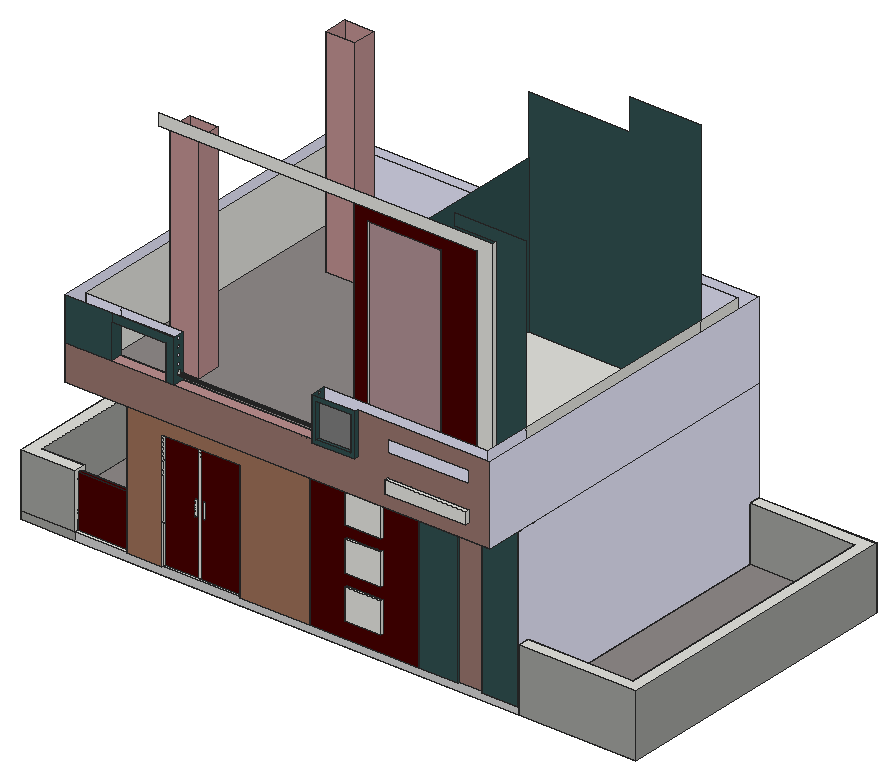
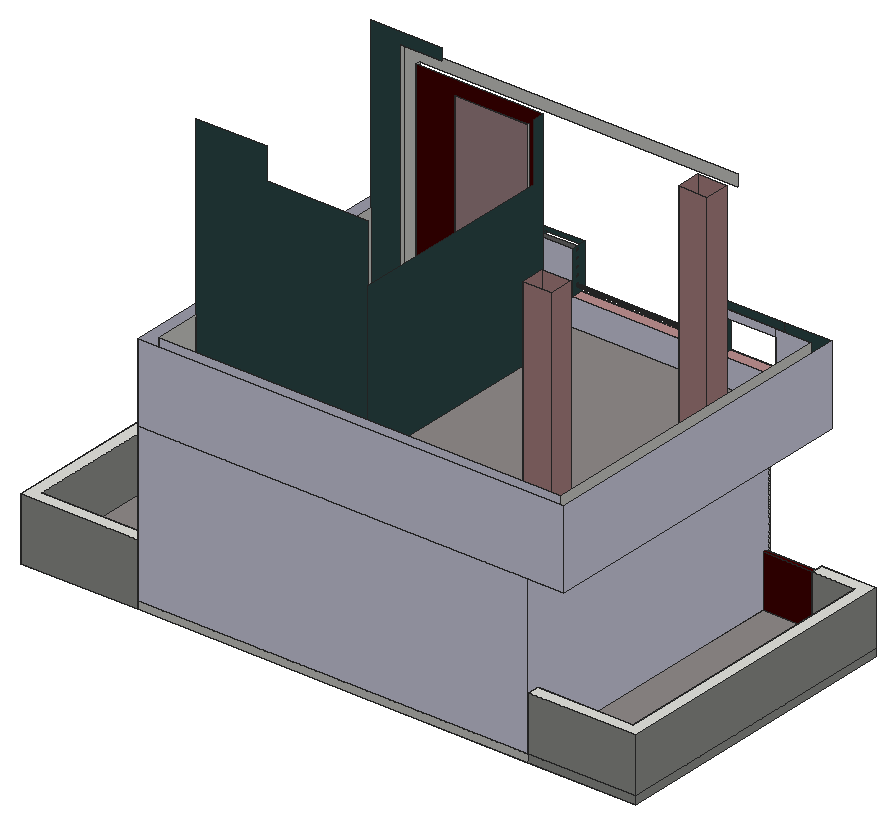
# SketchUp Ruby script. Lengths in inches.
U = 1.inch
M = Sketchup.active_model
def pt(a) = Geom::Point3d.new(a.map { |v| v * U })
def face(e, loops, mat)
  f = e.add_face(loops[0].map { |a| pt(a) })
  loops[1..].each { |l| e.add_face(l.map { |a| pt(a) }).erase! }
  f.material = f.back_material = mat if mat
  f
end
# faces: each face lists its corners as indices into pts; further lists are holes
def faces(e, pts, list, mat = nil) = list.each { |f| face(e, (f[0].is_a?(Array) ? f : [f]).map { |l| l.map { |i| pts[i] } }, mat) }
# xy, xz, yz: faces in a plane at the given z, y or x. An outline is a flat list of corners, or four numbers for a rectangle; further outlines are holes
def ring(l) = l.size == 4 ? [[l[0], l[1]], [l[2], l[1]], [l[2], l[3]], [l[0], l[3]]] : l.each_slice(2).to_a
def flat(e, list, mat, &to3) = list.each { |f| face(e, (f[0].is_a?(Array) ? f : [f]).map { |l| ring(l).map { |u, v| to3.(u, v) } }, mat) }
def xy(e, z, list, mat = nil) = flat(e, list, mat) { |x, y| [x, y, z] }
def xz(e, y, list, mat = nil) = flat(e, list, mat) { |x, z| [x, y, z] }
def yz(e, x, list, mat = nil) = flat(e, list, mat) { |y, z| [x, y, z] }
def lines(e, pts, list) = list.each { |a, b| e.add_line(pt(pts[a]), pt(pts[b])) }
# prism: a flat outline (further loops are holes) pulled along v
def prism(e, loops, v, mat = nil)
  f = face(e, loops, mat); d = Geom::Vector3d.new(v.map { |x| x * U })
  f.pushpull(f.normal.samedirection?(d) ? d.length : -d.length)
end
def box(e, o, s, mat = nil) = prism(e, [[o, [o[0] + s[0], o[1], o[2]], [o[0] + s[0], o[1] + s[1], o[2]], [o[0], o[1] + s[1], o[2]]]], [0, 0, s[2]], mat)
def at(x, y, z, deg = 0) = Geom::Transformation.translation(pt([x, y, z])) * Geom::Transformation.rotation(ORIGIN, Z_AXIS, deg.degrees)
def axes(o, x, y, z) = Geom::Transformation.new([*x, 0, *y, 0, *z, 0, *pt(o).to_a, 1])
def part(name) = M.definitions.add(name)
# library, detail: a bought-in or finely detailed component or shape, given as its bounding box
def library(name, o, s) = part(name).tap { |d| box(d.entities, o, s) }
def detail(e, o, s) = box(e.add_group.entities, o, s)
def put(e, d, t, mat = nil) = e.add_instance(d, t).tap { |i| i.material = mat if mat }
def group(e, t, mat = nil) = e.add_group.tap { |g| g.transformation = t; g.material = mat if mat }.entities
root = M.entities
M.materials.add("[0022_Maroon]").color = [71, 0, 0]
M.materials.add("[0040_Peru]").color = [150, 115, 108]
M.materials.add("[0078_DarkSlateGray]").color = [47, 79, 79]
M.materials.add("[0116_Lavender]").color = [230, 230, 250]
M.materials.add("[0118_Thistle]").color = [216, 191, 216]
M.materials.add("[0119_RosyBrown]").color = [188, 143, 143]
M.materials.add("[Carrera Marble]").color = [207, 207, 207]
M.materials.add("[Checker Plate]").color = [173, 142, 146]
M.materials.add("[Cladding Siding Tan]").color = [155, 110, 87]
M.materials.add("[Concrete Block 8x8 Gray]").color = [159, 160, 156]
M.materials.add("[Crushed Rock Gravel]").color = [124, 124, 124]
M.materials.add("[Stone Marble]").color = [143, 138, 136]
xy(root,0,[[0,60,165,522],[165,60,765,522],[765,60,945,522]])
xy(root,12,[[165,58,218.1875,60],[338.1875,58,446.1875,60],[446.1875,58,614.1875,60],[0,60,0,522,165,522,165,504,18,504,18,78,84,78,84,60],[84,60,165,65.6],
  [165,60,165,210,183,210,183,78,218.1875,78,218.1875,60],[338.1875,60,338.1875,78,747,78,747,210,765,210,765,60],[218.1875,64.63,338.1875,73.27],[84,65.6,165,71.35],[218.1875,73.27,338.1875,78],
  [183,78,747,210],[165,210,291.55,222],[291.55,210,388.24,214.18],[388.24,210,765,222],[291.55,214.18,388.24,218.54],
  [291.55,218.54,388.24,222],[165,222,165,522,765,522,765,222,753,222,753,321,527.52,321,527.52,330,600,330,600,432.82,609,432.82,609,330,753,330,753,510,609,510,609,487.39,600,487.39,600,510,366,510,366,330,454.54,330,454.54,321,258.23,321,258.23,330,357,330,357,510,177,510,177,330,199.29,330,199.29,321,177,321,177,222],[177,222,753,222,753,321,527.52,321,527.52,330,454.54,330,454.54,321,258.23,321,258.23,330,199.29,330,199.29,321,177,321],[177,330,357,510],[366,330,600,330,600,432.82,609,432.82,609,487.39,600,487.39,600,510,366,510],
  [609,330,753,510]])
xy(root,12,[[614.1875,58,674.1875,60],[710.1875,58,765,60]],"[0078_DarkSlateGray]")
xy(root,12,[[218.1875,60,338.1875,64.63]],"[Carrera Marble]")
xy(root,12,[[84,71.35,165,71.35,165,504,18,504,18,78,84,78],[765,78,927,504]],"[Stone Marble]")
xy(root,38.73,[[503.09,55,557.71,58]])
xy(root,86.3,[[503.09,55,557.71,58]])
xy(root,92.125,[[84,65.6,165,71.35]],"[0022_Maroon]")
xy(root,96,[[0,60,84,60,84,78,18,78,18,504,165,504,165,522,0,522],[765,60,945,60,945,522,765,522,765,504,927,504,927,78,765,78]])
xy(root,105.11,[[503.09,55,557.71,58]])
xy(root,142.5,[[600,432.82,609,487.39]])
xy(root,152.67,[[503.09,55,557.71,58]])
xy(root,157,[[199.29,321,258.23,330],[454.54,321,527.52,330]])
xy(root,168.44,[[291.55,210,388.24,214.18],[291.55,214.18,388.24,218.54],[291.55,218.54,388.24,222]])
xy(root,171.67,[[503.09,55,557.71,58]])
xy(root,193.9375,[[218.1875,58,338.1875,60],[218.1875,60,338.1875,64.63],[218.1875,64.63,338.1875,73.27],[218.1875,73.27,338.1875,78]])
xy(root,219.23,[[503.09,55,557.71,58]])
xy(root,252,[[139.72,26.33,136.64,26.86,133.79,28.17,131.38,30.17,129.58,32.73,128.49,35.67,128.21,38.79,128.74,41.88,130.05,44.72,132.06,47.13,134.62,48.9375,137.56,50.02,140.68,50.31,143.76,49.77,146.61,48.46,149.01,46.46,150.82,43.9,151.9,40.96,152.19,37.84,151.66,34.75,150.35,31.91,148.34,29.5,145.78,27.69,142.84,26.61],[230.54,26.33,227.45,26.86,224.6,28.17,222.2,30.17,220.39,32.73,219.31,35.67,219.02,38.79,219.55,41.88,220.87,44.72,222.87,47.13,225.43,48.9375,228.37,50.02,231.49,50.31,234.58,49.77,237.42,48.46,239.83,46.46,241.63,43.9,242.72,40.96,243,37.84,242.47,34.75,241.16,31.91,239.15,29.5,236.6,27.69,233.66,26.61],[333.47,26.33,330.39,26.86,327.54,28.17,325.13,30.17,323.33,32.73,322.24,35.67,321.96,38.79,322.49,41.88,323.8,44.72,325.81,47.13,328.37,48.9375,331.31,50.02,334.43,50.31,337.51,49.77,340.36,48.46,342.76,46.46,344.57,43.9,345.65,40.96,345.94,37.84,345.41,34.75,344.1,31.91,342.09,29.5,339.53,27.69,336.59,26.61],[453.47,26.33,450.39,26.86,447.54,28.17,445.13,30.17,443.33,32.73,442.24,35.67,441.96,38.79,442.49,41.88,443.8,44.72,445.81,47.13,448.37,48.9375,451.31,50.02,454.43,50.31,457.51,49.77,460.36,48.46,462.76,46.46,464.57,43.9,465.65,40.96,465.94,37.84,465.41,34.75,464.1,31.91,462.09,29.5,459.53,27.69,456.59,26.61],[573.47,26.33,570.39,26.86,567.54,28.17,565.13,30.17,563.33,32.73,562.24,35.67,561.96,38.79,562.49,41.88,563.8,44.72,565.81,47.13,568.37,48.9375,571.31,50.02,574.43,50.31,577.51,49.77,580.36,48.46,582.76,46.46,584.57,43.9,585.65,40.96,585.94,37.84,585.41,34.75,584.1,31.91,582.09,29.5,579.53,27.69,576.59,26.61],
  [693.47,26.33,690.39,26.86,687.54,28.17,685.13,30.17,683.33,32.73,682.24,35.67,681.96,38.79,682.49,41.88,683.8,44.72,685.81,47.13,688.37,48.9375,691.31,50.02,694.43,50.31,697.51,49.77,700.36,48.46,702.76,46.46,704.57,43.9,705.65,40.96,705.94,37.84,705.41,34.75,704.1,31.91,702.09,29.5,699.53,27.69,696.59,26.61],[165,58,218.1875,60],[218.1875,58,338.1875,60],[338.1875,58,446.1875,60],[446.1875,58,614.1875,60],
  [614.1875,58,674.1875,60],[710.1875,58,765,60],[165,60,165,210,183,210,183,78,218.1875,78,218.1875,60],[218.1875,60,338.1875,78],[338.1875,60,338.1875,78,747,78,747,210,765,210,765,60],
  [183,78,747,210],[136.96,95.37,133.87,95.86,131.01,97.13,128.57,99.11,126.73,101.64,125.61,104.57,125.29,107.68,125.78,110.78,127.05,113.64,129.03,116.07,131.5625,117.91,134.49,119.03,137.6,119.36,140.7,118.86,143.56,117.59,145.99,115.62,147.83,113.08,148.95,110.15,149.28,107.04,148.79,103.95,147.51,101.08,145.54,98.65,143,96.8125,140.08,95.69],[165,210,765,222],[136.96,215.37,133.87,215.86,131.01,217.13,128.57,219.11,126.73,221.64,125.61,224.57,125.29,227.68,125.78,230.78,127.05,233.64,129.03,236.07,131.5625,237.91,134.49,239.03,137.6,239.36,140.7,238.86,143.56,237.59,145.99,235.62,147.83,233.08,148.95,230.15,149.28,227.04,148.79,223.95,147.51,221.08,145.54,218.65,143,216.8125,140.08,215.69],[165,222,165,522,765,522,765,222,753,222,753,321,609,321,609,330,753,330,753,510,609,510,609,321,600,321,600,510,366,510,366,321,357,321,357,510,177,510,177,330,357,330,357,321,177,321,177,222],
  [177,222,177,321,357,321,357,330,177,330,177,510,357,510,357,321,366,321,366,510,600,510,600,321,609,321,609,510,753,510,753,330,609,330,609,321,753,321,753,222],[366,321,600,330],[136.96,335.37,133.87,335.86,131.01,337.13,128.57,339.11,126.73,341.64,125.61,344.57,125.29,347.68,125.78,350.78,127.05,353.64,129.03,356.07,131.5625,357.91,134.49,359.03,137.6,359.36,140.7,358.86,143.56,357.59,145.99,355.62,147.83,353.08,148.95,350.15,149.28,347.04,148.79,343.95,147.51,341.08,145.54,338.65,143,336.8125,140.08,335.69],[136.96,455.37,133.87,455.86,131.01,457.13,128.57,459.11,126.73,461.64,125.61,464.57,125.29,467.68,125.78,470.78,127.05,473.64,129.03,476.07,131.5625,477.91,134.49,479.03,137.6,479.36,140.7,478.86,143.56,477.59,145.99,475.62,147.83,473.08,148.95,470.15,149.28,467.04,148.79,463.95,147.51,461.08,145.54,458.65,143,456.8125,140.08,455.69]])
xy(root,252,[[[111,6,111,522,165,522,165,58,674.1875,58,674.1875,60,710.1875,60,710.1875,58,765,58,765,6],[136.96,335.37,140.08,335.69,143,336.8125,145.54,338.65,147.51,341.08,148.79,343.95,149.28,347.04,148.95,350.15,147.83,353.08,145.99,355.62,143.56,357.59,140.7,358.86,137.6,359.36,134.49,359.03,131.5625,357.91,129.03,356.07,127.05,353.64,125.78,350.78,125.29,347.68,125.61,344.57,126.73,341.64,128.57,339.11,131.01,337.13,133.87,335.86],[136.96,215.37,140.08,215.69,143,216.8125,145.54,218.65,147.51,221.08,148.79,223.95,149.28,227.04,148.95,230.15,147.83,233.08,145.99,235.62,143.56,237.59,140.7,238.86,137.6,239.36,134.49,239.03,131.5625,237.91,129.03,236.07,127.05,233.64,125.78,230.78,125.29,227.68,125.61,224.57,126.73,221.64,128.57,219.11,131.01,217.13,133.87,215.86],[136.96,95.37,140.08,95.69,143,96.8125,145.54,98.65,147.51,101.08,148.79,103.95,149.28,107.04,148.95,110.15,147.83,113.08,145.99,115.62,143.56,117.59,140.7,118.86,137.6,119.36,134.49,119.03,131.5625,117.91,129.03,116.07,127.05,113.64,125.78,110.78,125.29,107.68,125.61,104.57,126.73,101.64,128.57,99.11,131.01,97.13,133.87,95.86],[230.54,26.33,233.66,26.61,236.6,27.69,239.15,29.5,241.16,31.91,242.47,34.75,243,37.84,242.72,40.96,241.63,43.9,239.83,46.46,237.42,48.46,234.58,49.77,231.49,50.31,228.37,50.02,225.43,48.9375,222.87,47.13,220.87,44.72,219.55,41.88,219.02,38.79,219.31,35.67,220.39,32.73,222.2,30.17,224.6,28.17,227.45,26.86],[333.47,26.33,336.59,26.61,339.53,27.69,342.09,29.5,344.1,31.91,345.41,34.75,345.94,37.84,345.65,40.96,344.57,43.9,342.76,46.46,340.36,48.46,337.51,49.77,334.43,50.31,331.31,50.02,328.37,48.9375,325.81,47.13,323.8,44.72,322.49,41.88,321.96,38.79,322.24,35.67,323.33,32.73,325.13,30.17,327.54,28.17,330.39,26.86],[453.47,26.33,456.59,26.61,459.53,27.69,462.09,29.5,464.1,31.91,465.41,34.75,465.94,37.84,465.65,40.96,464.57,43.9,462.76,46.46,460.36,48.46,457.51,49.77,454.43,50.31,451.31,50.02,448.37,48.9375,445.81,47.13,443.8,44.72,442.49,41.88,441.96,38.79,442.24,35.67,443.33,32.73,445.13,30.17,447.54,28.17,450.39,26.86],[573.47,26.33,576.59,26.61,579.53,27.69,582.09,29.5,584.1,31.91,585.41,34.75,585.94,37.84,585.65,40.96,584.57,43.9,582.76,46.46,580.36,48.46,577.51,49.77,574.43,50.31,571.31,50.02,568.37,48.9375,565.81,47.13,563.8,44.72,562.49,41.88,561.96,38.79,562.24,35.67,563.33,32.73,565.13,30.17,567.54,28.17,570.39,26.86],[693.47,26.33,696.59,26.61,699.53,27.69,702.09,29.5,704.1,31.91,705.41,34.75,705.94,37.84,705.65,40.96,704.57,43.9,702.76,46.46,700.36,48.46,697.51,49.77,694.43,50.31,691.31,50.02,688.37,48.9375,685.81,47.13,683.8,44.72,682.49,41.88,681.96,38.79,682.24,35.67,683.33,32.73,685.13,30.17,687.54,28.17,690.39,26.86],[139.72,26.33,142.84,26.61,145.78,27.69,148.34,29.5,150.35,31.91,151.66,34.75,152.19,37.84,151.9,40.96,150.82,43.9,149.01,46.46,146.61,48.46,143.76,49.77,140.68,50.31,137.56,50.02,134.62,48.9375,132.06,47.13,130.05,44.72,128.74,41.88,128.21,38.79,128.49,35.67,129.58,32.73,131.38,30.17,133.79,28.17,136.64,26.86],[136.96,455.37,140.08,455.69,143,456.8125,145.54,458.65,147.51,461.08,148.79,463.95,149.28,467.04,148.95,470.15,147.83,473.08,145.99,475.62,143.56,477.59,140.7,478.86,137.6,479.36,134.49,479.03,131.5625,477.91,129.03,476.07,127.05,473.64,125.78,470.78,125.29,467.68,125.61,464.57,126.73,461.64,128.57,459.11,131.01,457.13,133.87,455.86]]],"[0118_Thistle]")
xy(root,264,[[677.8125,90,677.8125,96,483,96,483,432,747,432,747,96,701.8125,96,701.8125,90],[201,96,245.25,133.3125],[201,394.6875,245.25,432]])
xy(root,264,[[[129,24,747,24,747,96,701.8125,96,701.8125,90,677.8125,90,677.8125,96,483,96,483,432,747,432,747,504,129,504],[201,394.6875,245.25,432],[201,96,245.25,133.3125]]],"[Stone Marble]")
xy(root,275.13,[[607.99,0,731.55,6]])
xy(root,286.07,[[505.07,96,616.93,98]])
xy(root,294.2,[[607.99,0,731.55,6]])
xy(root,306,[[495,0,561,6],[267,6,279,24]])
xy(root,306,[[183,6,267,24],[279,6,495,24]],"[0119_RosyBrown]")
xy(root,312.125,[[501.125,0,554.875,6]],"[0078_DarkSlateGray]")
xz(root,0,[[607.99,275.13,731.55,294.2]])
xz(root,0,[[[495,306,561,372],[501.125,312.125,554.875,365.875]]],"[0078_DarkSlateGray]")
xz(root,6,[[607.99,275.13,731.55,294.2]])
xz(root,6,[[[111,252,765,252,765,372,561,372,561,306,111,306],[607.99,329.13,731.55,348.2],[607.99,275.13,731.55,294.2]]],"[0040_Peru]")
xz(root,6,[[111,306,183,372],[267,306,279,306,279,372,183,372,183,360,267,360]],"[0078_DarkSlateGray]")
xz(root,6,[[501.125,312.125,554.875,365.875]],"[Crushed Rock Gravel]")
xz(root,24,[[129,264,129,372,183,372,183,306,495,306,495,372,747,372,747,264],[267,306,267,360,183,360,183,372,279,372,279,306]],"[0116_Lavender]")
xz(root,55,[[503.09,38.73,557.71,86.3],[503.09,105.11,557.71,152.67],[503.09,171.67,557.71,219.23]])
xz(root,58,[[503.09,38.73,557.71,86.3],[503.09,105.11,557.71,152.67],[503.09,171.67,557.71,219.23]])
xz(root,58,[[[446.1875,12,614.1875,252],[503.09,171.67,557.71,219.23],[503.09,105.11,557.71,152.67],[503.09,38.73,557.71,86.3]]],"[0022_Maroon]")
xz(root,58,[[614.1875,12,674.1875,252],[710.1875,12,765,252]],"[0078_DarkSlateGray]")
xz(root,58,[[165,12,218.1875,12,218.1875,193.9375,338.1875,193.9375,338.1875,12,446.1875,12,446.1875,252,165,252]],"[Cladding Siding Tan]")
xz(root,60,[[165,12,165,252,446.1875,252,446.1875,12,338.1875,12,338.1875,193.9375,218.1875,193.9375,218.1875,12],[446.1875,12,614.1875,252],[614.1875,12,674.1875,252],[710.1875,12,765,252]])
xz(root,60,[[674.1875,12,710.1875,252]],"[0040_Peru]")
xz(root,60,[[84,0,765,12]],"[Carrera Marble]")
xz(root,60,[[0,0,84,12],[765,0,945,96],[0,12,84,96]],"[Concrete Block 8x8 Gray]")
xz(root,64.63,[[270.93,12,272.88,193.9375],[264.42,94.01,268.42,120.19],[276.42,94.01,280.42,120.19]])
xz(root,64.63,[[[218.1875,12,270.93,193.9375],[264.42,94.01,268.42,120.19]],[[272.88,12,338.1875,193.9375],[276.42,94.01,280.42,120.19]]],"[0022_Maroon]")
xz(root,65.6,[[84,12,165,92.125]],"[0022_Maroon]")
xz(root,71.35,[[84,12,165,92.125]],"[0022_Maroon]")
xz(root,73.27,[[218.1875,12,338.1875,193.9375]])
xz(root,78,[[183,12,218.1875,252],[338.1875,12,747,252],[218.1875,193.9375,338.1875,252]])
xz(root,78,[[18,12,84,96],[765,12,927,96]],"[Concrete Block 8x8 Gray]")
xz(root,90,[[677.8125,264,701.8125,264,701.8125,612,189,612,189,594,677.8125,594]])
xz(root,96,[[[483,264,677.8125,594],[505.07,286.07,616.93,571.93]]],"[0022_Maroon]")
xz(root,96,[[701.8125,264,747,264,747,630,639,630,639,612,701.8125,612]],"[0078_DarkSlateGray]")
xz(root,96,[[201,264,245.25,594]],"[0119_RosyBrown]")
xz(root,98,[[505.07,286.07,616.93,571.93]],"[Checker Plate]")
xz(root,133.3125,[[201,264,245.25,594]],"[0119_RosyBrown]")
xz(root,210,[[183,12,291.55,12,291.55,168.44,388.24,168.44,388.24,12,747,12,747,252,183,252]])
xz(root,214.18,[[291.55,12,388.24,168.44]])
xz(root,218.54,[[291.55,12,388.24,168.44]])
xz(root,222,[[177,12,177,252,753,252,753,12,388.24,12,388.24,168.44,291.55,168.44,291.55,12]])
xz(root,321,[[177,12,199.29,12,199.29,157,258.23,157,258.23,12,357,12,357,252,177,252],[357,12,366,252],[366,12,454.54,12,454.54,157,527.52,157,527.52,12,600,12,600,252,366,252],[600,12,609,252],[609,12,753,252]])
xz(root,330,[[177,12,177,252,357,252,357,12,258.23,12,258.23,157,199.29,157,199.29,12],[366,12,366,252,600,252,600,12,527.52,12,527.52,157,454.54,157,454.54,12],[609,12,753,252]])
xz(root,394.6875,[[201,264,245.25,594]],"[0119_RosyBrown]")
xz(root,432,[[483,264,483,594,639,594,639,642,747,642,747,264]],"[0078_DarkSlateGray]")
xz(root,432,[[201,264,245.25,594]],"[0119_RosyBrown]")
xz(root,432.82,[[600,12,609,142.5]])
xz(root,487.39,[[600,12,609,142.5]])
xz(root,504,[[129,264,747,372]],"[0116_Lavender]")
xz(root,504,[[18,12,165,96],[765,12,927,96]],"[Concrete Block 8x8 Gray]")
xz(root,510,[[177,12,357,252],[366,12,600,252],[609,12,753,252]])
xz(root,522,[[165,0,765,12]])
xz(root,522,[[165,12,765,252],[111,252,765,372]],"[0116_Lavender]")
xz(root,522,[[0,0,165,12],[765,0,945,96],[0,12,165,96]],"[Concrete Block 8x8 Gray]")
yz(root,0,[[60,0,522,12],[60,12,522,96]],"[Concrete Block 8x8 Gray]")
yz(root,18,[[78,12,504,96]],"[Concrete Block 8x8 Gray]")
yz(root,84,[[60,12,65.6,12,65.6,92.125,71.35,92.125,71.35,12,78,12,78,96,60,96],[65.6,12,71.35,92.125]])
yz(root,111,[[6,252,522,372]],"[0116_Lavender]")
yz(root,129,[[24,264,504,372]])
yz(root,165,[[58,12,60,252],[504,12,522,96]])
yz(root,165,[[60,12,60,252,522,252,522,96,504,96,504,12,71.35,12,71.35,92.125,65.6,92.125,65.6,12]],"[0116_Lavender]")
yz(root,177,[[222,12,321,252],[330,12,510,252]])
yz(root,183,[[78,12,210,252]])
yz(root,183,[[6,306,24,360]],"[0078_DarkSlateGray]")
yz(root,199.29,[[321,12,330,157]])
yz(root,201,[[96,264,133.3125,594],[394.6875,264,432,594]],"[0119_RosyBrown]")
yz(root,218.1875,[[58,12,60,193.9375],[60,12,64.63,193.9375],[64.63,12,73.27,193.9375],[73.27,12,78,193.9375]])
yz(root,245.25,[[96,264,133.3125,594],[394.6875,264,432,594]],"[0119_RosyBrown]")
yz(root,258.23,[[321,12,330,157]])
yz(root,267,[[6,306,24,360]],"[0078_DarkSlateGray]")
yz(root,279,[[15,316.75,14.22,316.85,13.5,317.15,12.88,317.625,12.4,318.25,12.1,318.97,12,319.75,12.1,320.52,12.4,321.25,12.88,321.87,13.5,322.34,14.22,322.64,15,322.75,15.78,322.64,16.5,322.34,17.12,321.87,17.6,321.25,17.9,320.52,18,319.75,17.9,318.97,17.6,318.25,17.12,317.625,16.5,317.15,15.78,316.85]])
yz(root,279,[[[6,306,24,372],[15,316.75,14.22,316.85,13.5,317.15,12.88,317.625,12.4,318.25,12.1,318.97,12,319.75,12.1,320.52,12.4,321.25,12.88,321.87,13.5,322.34,14.22,322.64,15,322.75,15.78,322.64,16.5,322.34,17.12,321.87,17.6,321.25,17.9,320.52,18,319.75,17.9,318.97,17.6,318.25,17.12,317.625,16.5,317.15,15.78,316.85],[15,340.75,14.22,340.85,13.5,341.15,12.88,341.625,12.4,342.25,12.1,342.97,12,343.75,12.1,344.52,12.4,345.25,12.88,345.87,13.5,346.34,14.22,346.64,15,346.75,15.78,346.64,16.5,346.34,17.12,345.87,17.6,345.25,17.9,344.52,18,343.75,17.9,342.97,17.6,342.25,17.12,341.625,16.5,341.15,15.78,340.85],[15,328.75,14.22,328.85,13.5,329.15,12.88,329.625,12.4,330.25,12.1,330.97,12,331.75,12.1,332.52,12.4,333.25,12.88,333.87,13.5,334.34,14.22,334.64,15,334.75,15.78,334.64,16.5,334.34,17.12,333.87,17.6,333.25,17.9,332.52,18,331.75,17.9,330.97,17.6,330.25,17.12,329.625,16.5,329.15,15.78,328.85],[15,352.75,14.22,352.85,13.5,353.15,12.88,353.625,12.4,354.25,12.1,354.97,12,355.75,12.1,356.52,12.4,357.25,12.88,357.87,13.5,358.34,14.22,358.64,15,358.75,15.78,358.64,16.5,358.34,17.12,357.87,17.6,357.25,17.9,356.52,18,355.75,17.9,354.97,17.6,354.25,17.12,353.625,16.5,353.15,15.78,352.85],[15,364.75,14.22,364.85,13.5,365.15,12.88,365.625,12.4,366.25,12.1,366.97,12,367.75,12.1,368.52,12.4,369.25,12.88,369.87,13.5,370.34,14.22,370.64,15,370.75,15.78,370.64,16.5,370.34,17.12,369.87,17.6,369.25,17.9,368.52,18,367.75,17.9,366.97,17.6,366.25,17.12,365.625,16.5,365.15,15.78,364.85]]],"[0078_DarkSlateGray]")
yz(root,291.55,[[210,12,214.18,168.44],[214.18,12,218.54,168.44],[218.54,12,222,168.44]])
yz(root,338.1875,[[58,12,60,193.9375],[60,12,64.63,193.9375],[64.63,12,73.27,193.9375],[73.27,12,78,193.9375]])
yz(root,357,[[330,12,510,252]])
yz(root,366,[[330,12,510,252]])
yz(root,388.24,[[210,12,214.18,168.44],[214.18,12,218.54,168.44],[218.54,12,222,168.44]])
yz(root,446.1875,[[58,12,60,252]])
yz(root,454.54,[[321,12,330,157]])
yz(root,483,[[96,264,96,594,114,594,114,504,432,504,432,264]],"[0078_DarkSlateGray]")
yz(root,495,[[[0,306,24,372],[15,316.75,15.78,316.85,16.5,317.15,17.12,317.625,17.6,318.25,17.9,318.97,18,319.75,17.9,320.52,17.6,321.25,17.12,321.87,16.5,322.34,15.78,322.64,15,322.75,14.22,322.64,13.5,322.34,12.88,321.87,12.4,321.25,12.1,320.52,12,319.75,12.1,318.97,12.4,318.25,12.88,317.625,13.5,317.15,14.22,316.85],[15,328.75,15.78,328.85,16.5,329.15,17.12,329.625,17.6,330.25,17.9,330.97,18,331.75,17.9,332.52,17.6,333.25,17.12,333.87,16.5,334.34,15.78,334.64,15,334.75,14.22,334.64,13.5,334.34,12.88,333.87,12.4,333.25,12.1,332.52,12,331.75,12.1,330.97,12.4,330.25,12.88,329.625,13.5,329.15,14.22,328.85],[15,340.75,15.78,340.85,16.5,341.15,17.12,341.625,17.6,342.25,17.9,342.97,18,343.75,17.9,344.52,17.6,345.25,17.12,345.87,16.5,346.34,15.78,346.64,15,346.75,14.22,346.64,13.5,346.34,12.88,345.87,12.4,345.25,12.1,344.52,12,343.75,12.1,342.97,12.4,342.25,12.88,341.625,13.5,341.15,14.22,340.85],[15,352.75,15.78,352.85,16.5,353.15,17.12,353.625,17.6,354.25,17.9,354.97,18,355.75,17.9,356.52,17.6,357.25,17.12,357.87,16.5,358.34,15.78,358.64,15,358.75,14.22,358.64,13.5,358.34,12.88,357.87,12.4,357.25,12.1,356.52,12,355.75,12.1,354.97,12.4,354.25,12.88,353.625,13.5,353.15,14.22,352.85],[15,364.75,15.78,364.85,16.5,365.15,17.12,365.625,17.6,366.25,17.9,366.97,18,367.75,17.9,368.52,17.6,369.25,17.12,369.87,16.5,370.34,15.78,370.64,15,370.75,14.22,370.64,13.5,370.34,12.88,369.87,12.4,369.25,12.1,368.52,12,367.75,12.1,366.97,12.4,366.25,12.88,365.625,13.5,365.15,14.22,364.85]]],"[0078_DarkSlateGray]")
yz(root,501.125,[[0,312.125,6,365.875]],"[0078_DarkSlateGray]")
yz(root,503.09,[[55,38.73,58,86.3],[55,105.11,58,152.67],[55,171.67,58,219.23]])
yz(root,505.07,[[96,286.07,98,571.93]])
yz(root,527.52,[[321,12,330,157]])
yz(root,554.875,[[0,312.125,6,365.875]],"[0078_DarkSlateGray]")
yz(root,557.71,[[55,38.73,58,86.3],[55,105.11,58,152.67],[55,171.67,58,219.23]])
yz(root,561,[[0,306,6,372]],"[0078_DarkSlateGray]")
yz(root,600,[[330,12,330,252,510,252,510,12,487.39,12,487.39,142.5,432.82,142.5,432.82,12]])
yz(root,607.99,[[0,275.13,6,294.2]])
yz(root,609,[[330,12,432.82,12,432.82,142.5,487.39,142.5,487.39,12,510,12,510,252,330,252]])
yz(root,614.1875,[[58,12,60,252]])
yz(root,616.93,[[96,286.07,98,571.93]])
yz(root,674.1875,[[58,12,60,252]],"[0078_DarkSlateGray]")
yz(root,677.8125,[[90,264,96,594]])
yz(root,701.8125,[[90,264,96,612]])
yz(root,710.1875,[[58,12,60,252]])
yz(root,731.55,[[0,275.13,6,294.2]])
yz(root,747,[[78,12,210,252],[96,264,432,372],[432,264,504,372]])
yz(root,747,[[24,264,96,372]],"[0116_Lavender]")
yz(root,753,[[222,12,321,252],[330,12,510,252]])
yz(root,765,[[60,0,522,12],[60,12,78,96],[504,12,522,96]])
yz(root,765,[[58,12,60,96],[58,96,60,252]],"[0078_DarkSlateGray]")
yz(root,765,[[78,12,504,12,504,96,522,96,522,252,60,252,60,96,78,96],[6,252,522,372]],"[0116_Lavender]")
yz(root,927,[[78,12,504,96]],"[Concrete Block 8x8 Gray]")
yz(root,945,[[60,0,522,96]],"[Concrete Block 8x8 Gray]")
p = [[279,14.22,316.85],[279,15,316.75],[495,15,316.75],[495,14.22,316.85],[279,15.78,316.85],[495,15.78,316.85],
  [279,13.5,317.15],[495,13.5,317.15],[279,16.5,317.15],[495,16.5,317.15],[279,12.88,317.625],[495,12.88,317.625],
  [279,17.12,317.625],[495,17.12,317.625],[279,12.4,318.25],[495,12.4,318.25],[279,17.6,318.25],[495,17.6,318.25]]
faces(root,p,[[0,1,2,3],[1,4,5,2],[6,0,3,7],[4,8,9,5],[10,6,7,11],[8,12,13,9],[14,10,11,15],[12,16,17,13]])
